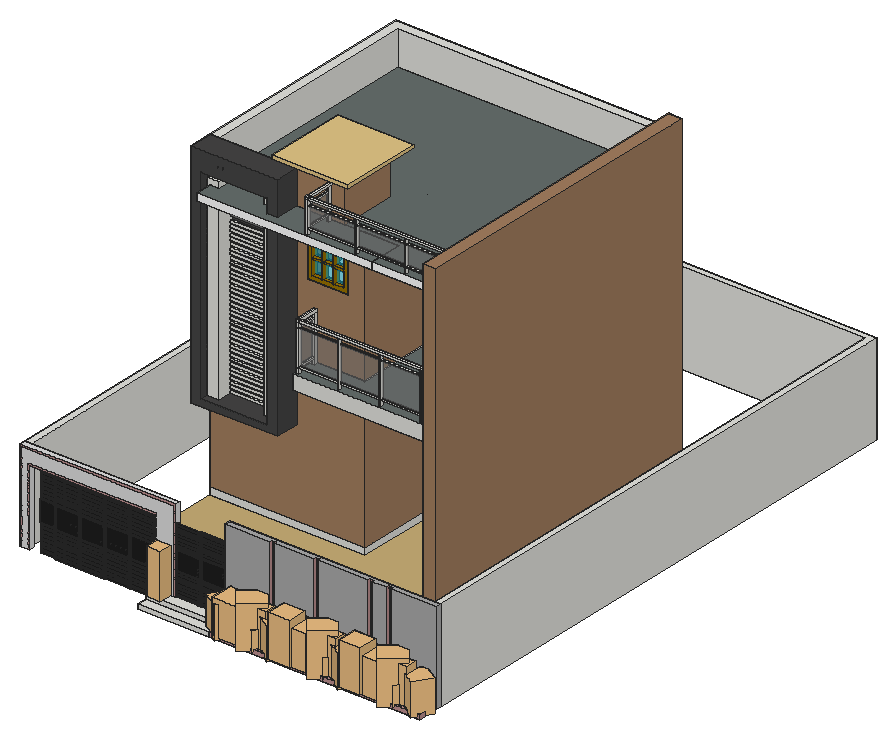
# SketchUp Ruby script. Lengths in inches.
U = 1.inch
M = Sketchup.active_model
def pt(a) = Geom::Point3d.new(a.map { |v| v * U })
def face(e, loops, mat)
  f = e.add_face(loops[0].map { |a| pt(a) })
  loops[1..].each { |l| e.add_face(l.map { |a| pt(a) }).erase! }
  f.material = f.back_material = mat if mat
  f
end
# faces: each face lists its corners as indices into pts; further lists are holes
def faces(e, pts, list, mat = nil) = list.each { |f| face(e, (f[0].is_a?(Array) ? f : [f]).map { |l| l.map { |i| pts[i] } }, mat) }
# xy, xz, yz: faces in a plane at the given z, y or x. An outline is a flat list of corners, or four numbers for a rectangle; further outlines are holes
def ring(l) = l.size == 4 ? [[l[0], l[1]], [l[2], l[1]], [l[2], l[3]], [l[0], l[3]]] : l.each_slice(2).to_a
def flat(e, list, mat, &to3) = list.each { |f| face(e, (f[0].is_a?(Array) ? f : [f]).map { |l| ring(l).map { |u, v| to3.(u, v) } }, mat) }
def xy(e, z, list, mat = nil) = flat(e, list, mat) { |x, y| [x, y, z] }
def xz(e, y, list, mat = nil) = flat(e, list, mat) { |x, z| [x, y, z] }
def yz(e, x, list, mat = nil) = flat(e, list, mat) { |y, z| [x, y, z] }
def lines(e, pts, list) = list.each { |a, b| e.add_line(pt(pts[a]), pt(pts[b])) }
# prism: a flat outline (further loops are holes) pulled along v
def prism(e, loops, v, mat = nil)
  f = face(e, loops, mat); d = Geom::Vector3d.new(v.map { |x| x * U })
  f.pushpull(f.normal.samedirection?(d) ? d.length : -d.length)
end
def box(e, o, s, mat = nil) = prism(e, [[o, [o[0] + s[0], o[1], o[2]], [o[0] + s[0], o[1] + s[1], o[2]], [o[0], o[1] + s[1], o[2]]]], [0, 0, s[2]], mat)
def at(x, y, z, deg = 0) = Geom::Transformation.translation(pt([x, y, z])) * Geom::Transformation.rotation(ORIGIN, Z_AXIS, deg.degrees)
def axes(o, x, y, z) = Geom::Transformation.new([*x, 0, *y, 0, *z, 0, *pt(o).to_a, 1])
def part(name) = M.definitions.add(name)
# library, detail: a bought-in or finely detailed component or shape, given as its bounding box
def library(name, o, s) = part(name).tap { |d| box(d.entities, o, s) }
def detail(e, o, s) = box(e.add_group.entities, o, s)
def put(e, d, t, mat = nil) = e.add_instance(d, t).tap { |i| i.material = mat if mat }
def group(e, t, mat = nil) = e.add_group.tap { |g| g.transformation = t; g.material = mat if mat }.entities
root = M.entities
M.materials.add("Color_008").color = [30, 30, 30]
M.materials.add("Material__1").color = [95, 70, 46]
M.materials.add("[0055_LightGoldenrodYellow]").color = [250, 250, 210]
M.materials.add("[0119_RosyBrown]").color = [188, 143, 143]
M.materials.add("[0130_Gainsboro]").color = [220, 220, 220]
M.materials.add("[0132_LightGray]").color = [169, 169, 169]
M.materials.add("[0134_DimGray]").color = [105, 105, 105]
M.materials.add("[0136_Charcoal]").color = [35, 35, 35]
M.materials.add("[Cladding Siding Tan]").color = [162, 126, 95]
M.materials.add("[Color D07]").color = [153, 114, 0]
M.materials.add("[Color E01]").color = [255, 255, 204]
M.materials.add("[Color M00]").color = [255, 255, 255]
M.materials.add("[Granite Dark Gray]").color = [69, 68, 68]
M.materials.add("[Metal Rusted]").color = [184, 117, 91]
M.materials.add("[Slate]").color = [102, 110, 108]
M.materials.add("[Stone Brushed Khaki]").color = [226, 197, 133]
M.materials.add("[Tile Limestone Multi]").color = [199, 173, 118]
M.materials.add("[Translucent Glass Gray]").color = [128, 128, 128]
M.materials["[Translucent Glass Gray]"].alpha = 0.5
M.materials.add("[Translucent Glass Tinted]").color = [8, 201, 241]
M.materials["[Translucent Glass Tinted]"].alpha = 0.48
M.materials.add("[Wood Bamboo]").color = [177, 105, 43]
M.materials.add("[Wood Floor Parquet]").color = [145, 89, 39]
c1 = part("Frame upright")
box(c1.entities,[0,0,0],[1.9,0.97,93.54])
c2 = part("Vertical picket")
box(c2.entities,[0,0,-2.03],[1.97,0.97,40.94])
c3 = part("Vertical picket \#1")
box(c3.entities,[2.95,0,-2.03],[0.99,0.97,40.94])
c4 = part("Slatted screen panel \#1")
put(c4.entities,c1,axes([87.6,0,0],[1,0,0],[0,1,0],[0,0,0.92593]),"Color_008")
put(c4.entities,c2,axes([48.6875,0,86.61],[0,0,-1],[0,1,0],[1,0,0]),"Color_008")
put(c4.entities,c1,axes([44.75,0,0],[1,0,0],[0,1,0],[0,0,0.92593]),"Color_008")
put(c4.entities,c3,axes([48.6875,0,87.11],[0,0,-1],[0,1,0],[1,0,0]),"[0134_DimGray]")
put(c4.entities,c2,axes([48.6875,0,82.68],[0,0,-1],[0,1,0],[1,0,0]),"Color_008")
put(c4.entities,c3,axes([48.6875,0,83.17],[0,0,-1],[0,1,0],[1,0,0]),"[0134_DimGray]")
put(c4.entities,c3,axes([48.6875,0,75.3],[0,0,-1],[0,1,0],[1,0,0]),"[0134_DimGray]")
put(c4.entities,c2,axes([48.6875,0,78.74],[0,0,-1],[0,1,0],[1,0,0]),"Color_008")
put(c4.entities,c2,axes([48.6875,0,74.8],[0,0,-1],[0,1,0],[1,0,0]),"Color_008")
put(c4.entities,c3,axes([48.6875,0,79.23],[0,0,-1],[0,1,0],[1,0,0]),"[0134_DimGray]")
put(c4.entities,c3,axes([48.6875,0,67.42],[0,0,-1],[0,1,0],[1,0,0]),"[0134_DimGray]")
put(c4.entities,c3,axes([48.6875,0,71.36],[0,0,-1],[0,1,0],[1,0,0]),"[0134_DimGray]")
put(c4.entities,c2,axes([48.6875,0,70.87],[0,0,-1],[0,1,0],[1,0,0]),"Color_008")
put(c4.entities,c2,axes([48.6875,0,66.93],[0,0,-1],[0,1,0],[1,0,0]),"Color_008")
put(c4.entities,c2,axes([48.6875,0,59.06],[0,0,-1],[0,1,0],[1,0,0]),"Color_008")
put(c4.entities,c2,axes([48.6875,0,62.99],[0,0,-1],[0,1,0],[1,0,0]),"Color_008")
put(c4.entities,c3,axes([48.6875,0,59.55],[0,0,-1],[0,1,0],[1,0,0]),"[0134_DimGray]")
put(c4.entities,c3,axes([48.6875,0,63.48],[0,0,-1],[0,1,0],[1,0,0]),"[0134_DimGray]")
put(c4.entities,c3,axes([48.6875,0,33.96],[0,0,-1],[0,1,0],[1,0,0]),"[0134_DimGray]")
put(c4.entities,c2,axes([48.6875,0,29.53],[0,0,-1],[0,1,0],[1,0,0]),"Color_008")
put(c4.entities,c3,axes([48.6875,0,30.02],[0,0,-1],[0,1,0],[1,0,0]),"[0134_DimGray]")
put(c4.entities,c2,axes([48.6875,0,25.59],[0,0,-1],[0,1,0],[1,0,0]),"Color_008")
put(c4.entities,c2,axes([48.6875,0,33.46],[0,0,-1],[0,1,0],[1,0,0]),"Color_008")
put(c4.entities,c3,axes([48.6875,0,26.08],[0,0,-1],[0,1,0],[1,0,0]),"[0134_DimGray]")
put(c4.entities,c2,axes([48.6875,0,13.78],[0,0,-1],[0,1,0],[1,0,0]),"Color_008")
put(c4.entities,c3,axes([48.6875,0,10.33],[0,0,-1],[0,1,0],[1,0,0]),"[0134_DimGray]")
put(c4.entities,c2,axes([48.6875,0,21.65],[0,0,-1],[0,1,0],[1,0,0]),"Color_008")
put(c4.entities,c2,axes([48.6875,0,5.91],[0,0,-1],[0,1,0],[1,0,0]),"Color_008")
put(c4.entities,c3,axes([48.6875,0,22.15],[0,0,-1],[0,1,0],[1,0,0]),"[0134_DimGray]")
put(c4.entities,c2,axes([48.6875,0,1.97],[0,0,-1],[0,1,0],[1,0,0]),"Color_008")
put(c4.entities,c2,axes([48.6875,0,9.84],[0,0,-1],[0,1,0],[1,0,0]),"Color_008")
put(c4.entities,c3,axes([48.6875,0,6.4],[0,0,-1],[0,1,0],[1,0,0]),"[0134_DimGray]")
put(c4.entities,c3,axes([48.6875,0,18.21],[0,0,-1],[0,1,0],[1,0,0]),"[0134_DimGray]")
put(c4.entities,c2,axes([48.6875,0,17.72],[0,0,-1],[0,1,0],[1,0,0]),"Color_008")
put(c4.entities,c3,axes([48.6875,0,14.27],[0,0,-1],[0,1,0],[1,0,0]),"[0134_DimGray]")
put(c4.entities,c2,axes([48.6875,0,49.7],[0,0,-1],[0,1,0],[1,0,0]),"Color_008")
put(c4.entities,c2,axes([48.6875,0,44.29],[0,0,-1],[0,1,0],[1,0,0]),"Color_008")
put(c4.entities,c2,axes([48.6875,0,38.88],[0,0,-1],[0,1,0],[1,0,0]),"Color_008")
put(c4.entities,c2,axes([48.6875,0,55.12],[0,0,-1],[0,1,0],[1,0,0]),"Color_008")
c5 = part("Infill panel")
box(c5.entities,[0,0,-1.97],[52.81,0.39,23.62])
c6 = part("Slatted screen panel")
p = [[42.85,0.97,43.31],[42.85,0.97,44.29]]
lines(c6.entities,p,[[0,1]])
put(c6.entities,c2,axes([3.9375,0,86.61],[0,0,-1],[0,1,0],[1,0,0]),"Color_008")
put(c6.entities,c1,axes([87.6,0,0],[1,0,0],[0,1,0],[0,0,0.92593]),"Color_008")
put(c6.entities,c2,axes([48.6875,0,86.61],[0,0,-1],[0,1,0],[1,0,0]),"Color_008")
put(c6.entities,c1,axes([0,0,0],[1,0,0],[0,1,0],[0,0,0.92593]),"Color_008")
put(c6.entities,c1,axes([42.85,0,0],[1,0,0],[0,1,0],[0,0,0.92593]),"Color_008")
put(c6.entities,c1,axes([44.75,0,0],[1,0,0],[0,1,0],[0,0,0.92593]),"Color_008")
put(c6.entities,c3,axes([3.9375,0,87.11],[0,0,-1],[0,1,0],[1,0,0]),"[0134_DimGray]")
put(c6.entities,c3,axes([48.6875,0,87.11],[0,0,-1],[0,1,0],[1,0,0]),"[0134_DimGray]")
put(c6.entities,c2,axes([48.6875,0,82.68],[0,0,-1],[0,1,0],[1,0,0]),"Color_008")
put(c6.entities,c3,axes([48.6875,0,83.17],[0,0,-1],[0,1,0],[1,0,0]),"[0134_DimGray]")
put(c6.entities,c3,axes([3.9375,0,83.17],[0,0,-1],[0,1,0],[1,0,0]),"[0134_DimGray]")
put(c6.entities,c2,axes([3.9375,0,82.68],[0,0,-1],[0,1,0],[1,0,0]),"Color_008")
put(c6.entities,c3,axes([48.6875,0,75.3],[0,0,-1],[0,1,0],[1,0,0]),"[0134_DimGray]")
put(c6.entities,c2,axes([48.6875,0,78.74],[0,0,-1],[0,1,0],[1,0,0]),"Color_008")
put(c6.entities,c2,axes([48.6875,0,74.8],[0,0,-1],[0,1,0],[1,0,0]),"Color_008")
put(c6.entities,c3,axes([48.6875,0,79.23],[0,0,-1],[0,1,0],[1,0,0]),"[0134_DimGray]")
put(c6.entities,c3,axes([3.9375,0,75.3],[0,0,-1],[0,1,0],[1,0,0]),"[0134_DimGray]")
put(c6.entities,c2,axes([3.9375,0,78.74],[0,0,-1],[0,1,0],[1,0,0]),"Color_008")
put(c6.entities,c3,axes([3.9375,0,79.23],[0,0,-1],[0,1,0],[1,0,0]),"[0134_DimGray]")
put(c6.entities,c2,axes([3.9375,0,74.8],[0,0,-1],[0,1,0],[1,0,0]),"Color_008")
put(c6.entities,c3,axes([48.6875,0,67.42],[0,0,-1],[0,1,0],[1,0,0]),"[0134_DimGray]")
put(c6.entities,c3,axes([3.9375,0,63.48],[0,0,-1],[0,1,0],[1,0,0]),"[0134_DimGray]")
put(c6.entities,c3,axes([48.6875,0,71.36],[0,0,-1],[0,1,0],[1,0,0]),"[0134_DimGray]")
put(c6.entities,c3,axes([3.9375,0,67.42],[0,0,-1],[0,1,0],[1,0,0]),"[0134_DimGray]")
put(c6.entities,c2,axes([3.9375,0,70.87],[0,0,-1],[0,1,0],[1,0,0]),"Color_008")
put(c6.entities,c2,axes([48.6875,0,70.87],[0,0,-1],[0,1,0],[1,0,0]),"Color_008")
put(c6.entities,c2,axes([48.6875,0,66.93],[0,0,-1],[0,1,0],[1,0,0]),"Color_008")
put(c6.entities,c2,axes([48.6875,0,59.06],[0,0,-1],[0,1,0],[1,0,0]),"Color_008")
put(c6.entities,c2,axes([3.9375,0,55.12],[0,0,-1],[0,1,0],[1,0,0]),"Color_008")
put(c6.entities,c2,axes([3.9375,0,62.99],[0,0,-1],[0,1,0],[1,0,0]),"Color_008")
put(c6.entities,c3,axes([3.9375,0,59.55],[0,0,-1],[0,1,0],[1,0,0]),"[0134_DimGray]")
put(c6.entities,c2,axes([3.9375,0,66.93],[0,0,-1],[0,1,0],[1,0,0]),"Color_008")
put(c6.entities,c2,axes([48.6875,0,62.99],[0,0,-1],[0,1,0],[1,0,0]),"Color_008")
put(c6.entities,c3,axes([48.6875,0,59.55],[0,0,-1],[0,1,0],[1,0,0]),"[0134_DimGray]")
put(c6.entities,c3,axes([48.6875,0,63.48],[0,0,-1],[0,1,0],[1,0,0]),"[0134_DimGray]")
put(c6.entities,c2,axes([3.9375,0,59.06],[0,0,-1],[0,1,0],[1,0,0]),"Color_008")
put(c6.entities,c3,axes([3.9375,0,71.36],[0,0,-1],[0,1,0],[1,0,0]),"[0134_DimGray]")
put(c6.entities,c3,axes([3.9375,0,33.96],[0,0,-1],[0,1,0],[1,0,0]),"[0134_DimGray]")
put(c6.entities,c3,axes([48.6875,0,33.96],[0,0,-1],[0,1,0],[1,0,0]),"[0134_DimGray]")
put(c6.entities,c2,axes([3.9375,0,29.53],[0,0,-1],[0,1,0],[1,0,0]),"Color_008")
put(c6.entities,c3,axes([3.9375,0,26.08],[0,0,-1],[0,1,0],[1,0,0]),"[0134_DimGray]")
put(c6.entities,c2,axes([3.9375,0,33.46],[0,0,-1],[0,1,0],[1,0,0]),"Color_008")
put(c6.entities,c2,axes([48.6875,0,29.53],[0,0,-1],[0,1,0],[1,0,0]),"Color_008")
put(c6.entities,c3,axes([48.6875,0,30.02],[0,0,-1],[0,1,0],[1,0,0]),"[0134_DimGray]")
put(c6.entities,c2,axes([3.9375,0,25.59],[0,0,-1],[0,1,0],[1,0,0]),"Color_008")
put(c6.entities,c2,axes([48.6875,0,25.59],[0,0,-1],[0,1,0],[1,0,0]),"Color_008")
put(c6.entities,c2,axes([48.6875,0,33.46],[0,0,-1],[0,1,0],[1,0,0]),"Color_008")
put(c6.entities,c2,axes([3.9375,0,49.7],[0,0,-1],[0,1,0],[1,0,0]),"Color_008")
put(c6.entities,c3,axes([48.6875,0,26.08],[0,0,-1],[0,1,0],[1,0,0]),"[0134_DimGray]")
put(c6.entities,c3,axes([3.9375,0,30.02],[0,0,-1],[0,1,0],[1,0,0]),"[0134_DimGray]")
put(c6.entities,c2,axes([3.9375,0,5.91],[0,0,-1],[0,1,0],[1,0,0]),"Color_008")
put(c6.entities,c2,axes([48.6875,0,13.78],[0,0,-1],[0,1,0],[1,0,0]),"Color_008")
put(c6.entities,c3,axes([48.6875,0,10.33],[0,0,-1],[0,1,0],[1,0,0]),"[0134_DimGray]")
put(c6.entities,c3,axes([3.9375,0,6.4],[0,0,-1],[0,1,0],[1,0,0]),"[0134_DimGray]")
put(c6.entities,c2,axes([3.9375,0,13.78],[0,0,-1],[0,1,0],[1,0,0]),"Color_008")
put(c6.entities,c2,axes([48.6875,0,21.65],[0,0,-1],[0,1,0],[1,0,0]),"Color_008")
put(c6.entities,c2,axes([48.6875,0,5.91],[0,0,-1],[0,1,0],[1,0,0]),"Color_008")
put(c6.entities,c3,axes([48.6875,0,22.15],[0,0,-1],[0,1,0],[1,0,0]),"[0134_DimGray]")
put(c6.entities,c2,axes([48.6875,0,1.97],[0,0,-1],[0,1,0],[1,0,0]),"Color_008")
put(c6.entities,c2,axes([48.6875,0,9.84],[0,0,-1],[0,1,0],[1,0,0]),"Color_008")
put(c6.entities,c3,axes([48.6875,0,6.4],[0,0,-1],[0,1,0],[1,0,0]),"[0134_DimGray]")
put(c6.entities,c2,axes([3.9375,0,9.84],[0,0,-1],[0,1,0],[1,0,0]),"Color_008")
put(c6.entities,c3,axes([3.9375,0,10.33],[0,0,-1],[0,1,0],[1,0,0]),"[0134_DimGray]")
put(c6.entities,c3,axes([3.9375,0,22.15],[0,0,-1],[0,1,0],[1,0,0]),"[0134_DimGray]")
put(c6.entities,c2,axes([3.9375,0,1.97],[0,0,-1],[0,1,0],[1,0,0]),"Color_008")
put(c6.entities,c3,axes([3.9375,0,18.21],[0,0,-1],[0,1,0],[1,0,0]),"[0134_DimGray]")
put(c6.entities,c3,axes([3.9375,0,14.27],[0,0,-1],[0,1,0],[1,0,0]),"[0134_DimGray]")
put(c6.entities,c2,axes([3.9375,0,21.65],[0,0,-1],[0,1,0],[1,0,0]),"Color_008")
put(c6.entities,c3,axes([48.6875,0,18.21],[0,0,-1],[0,1,0],[1,0,0]),"[0134_DimGray]")
put(c6.entities,c2,axes([3.9375,0,17.72],[0,0,-1],[0,1,0],[1,0,0]),"Color_008")
put(c6.entities,c2,axes([48.6875,0,17.72],[0,0,-1],[0,1,0],[1,0,0]),"Color_008")
put(c6.entities,c3,axes([48.6875,0,14.27],[0,0,-1],[0,1,0],[1,0,0]),"[0134_DimGray]")
put(c6.entities,c2,axes([3.9375,0,44.29],[0,0,-1],[0,1,0],[1,0,0]),"Color_008")
put(c6.entities,c2,axes([3.9375,0,38.88],[0,0,-1],[0,1,0],[1,0,0]),"Color_008")
put(c6.entities,c2,axes([48.6875,0,49.7],[0,0,-1],[0,1,0],[1,0,0]),"Color_008")
put(c6.entities,c2,axes([48.6875,0,44.29],[0,0,-1],[0,1,0],[1,0,0]),"Color_008")
put(c6.entities,c2,axes([48.6875,0,38.88],[0,0,-1],[0,1,0],[1,0,0]),"Color_008")
put(c6.entities,c2,axes([48.6875,0,55.12],[0,0,-1],[0,1,0],[1,0,0]),"Color_008")
c7 = part("Group\#19")
put(c7.entities,c5,axes([0,0,33.46],[0.82011,0,0],[0,1,0],[0,0,1]),"Color_008")
put(c7.entities,c6,axes([0,0.39,0],[0.96774,0,0],[0,1,0],[0,0,1]),"[0055_LightGoldenrodYellow]")
put(c7.entities,c5,axes([43.31,0,33.46],[0.82011,0,0],[0,1,0],[0,0,1]),"Color_008")
c8 = library("Areca palm plant",[0,0,0],[49.1,36.6,54.46])
c9 = library("Group\#74",[-84.69,-90.07,-0.36],[176.51,175.13,171.4])
c10 = library("Group\#130",[-7.34,-1.2,0],[38.67,35.81,49.04])
c11 = library("Group38\#2",[14.01,28.44,-23.43],[18.58,18.32,38.89])
c12 = library("Group20\#1",[-20.81,-17.08,3.79],[39.86,39.43,37.51])
c13 = library("Group\#39",[0,0,0],[39.23,38.16,78.77])
c14 = part("compound +++")
g1 = group(c14.entities,at(40.59,15.26,0))
g2 = group(g1,at(295.3,30.86,0),"[0132_LightGray]")
xy(g2,0,[[0,0,304.7,8]])
xy(g2,9,[[205.47,0,211.47,3]],"[0119_RosyBrown]")
xy(g2,9,[[64.54,0,70.54,3],[127.35,0,133.35,3],[232.97,0,238.97,3]],"[0136_Charcoal]")
xy(g2,84,[[0,0,64.54,0,64.54,3,70.54,3,70.54,0,127.35,0,127.35,3,133.35,3,133.35,0,205.47,0,205.47,3,211.47,3,211.47,0,232.97,0,232.97,3,238.97,3,238.97,0,304.7,0,304.7,8,0,8],[232.97,0,238.97,3]])
xz(g2,0,[[0,0,304.7,0,304.7,84,238.97,84,238.97,9,232.97,9,232.97,84,211.47,84,211.47,9,205.47,9,205.47,84,133.35,84,133.35,9,127.35,9,127.35,84,70.54,84,70.54,9,64.54,9,64.54,84,0,84]])
xz(g2,3,[[64.54,9,70.54,84],[127.35,9,133.35,84],[205.47,9,211.47,84],[232.97,9,238.97,84]],"[0119_RosyBrown]")
xz(g2,8,[[0,0,304.7,84]])
yz(g2,0,[[0,0,8,84]])
yz(g2,64.54,[[0,9,3,84]],"[0119_RosyBrown]")
yz(g2,70.54,[[0,9,3,84]],"[0119_RosyBrown]")
yz(g2,127.35,[[0,9,3,84]],"[0119_RosyBrown]")
yz(g2,133.35,[[0,9,3,84]],"[0119_RosyBrown]")
yz(g2,205.47,[[0,9,3,84]],"[0119_RosyBrown]")
yz(g2,211.47,[[0,9,3,84]],"[0119_RosyBrown]")
yz(g2,232.97,[[0,9,3,84]],"[0119_RosyBrown]")
yz(g2,238.97,[[0,9,3,84]],"[0119_RosyBrown]")
yz(g2,304.7,[[0,0,8,84]])
g3 = group(g1,at(0,30.86,0),"[0130_Gainsboro]")
xy(g3,0,[[0,0,13.34,8],[193.34,0,223.34,8]])
xy(g3,69,[[13.34,0,193.34,8]])
xy(g3,84,[[0,0,223.34,8]])
xz(g3,0,[[2,0,11.34,0,11.34,71,195.34,71,195.34,0,221.34,0,221.34,82,2,82]])
xz(g3,0,[[0,0,2,0,2,82,221.34,82,221.34,0,223.34,0,223.34,84,0,84],[11.34,0,13.34,0,13.34,69,193.34,69,193.34,0,195.34,0,195.34,71,11.34,71]],"[0119_RosyBrown]")
xz(g3,8,[[0,0,0,84,223.34,84,223.34,0,193.34,0,193.34,69,13.34,69,13.34,0]])
yz(g3,0,[[0,0,8,84]])
yz(g3,13.34,[[0,0,8,69]])
yz(g3,193.34,[[0,0,8,69]])
yz(g3,223.34,[[0,0,8,84]])
g4 = group(g1,at(13.34,31.16,0))
g5 = group(g4,at(13.67,1.64,0))
put(g5,c4,axes([-35.99,0.33,0],[0.80418,0,0],[0,0.83,0],[0,0,0.79664]),"[0055_LightGoldenrodYellow]")
put(g5,c5,axes([0,0,26.66],[0.68149,0,0],[0,0.83,0],[0,0,0.79664]),"Color_008")
g6 = group(g4,at(35.99,0,0))
put(g6,c7,axes([0,0,0],[0.83098,0,0],[0,0.83,0],[0,0,0.79664]))
put(g6,c7,axes([71.97,0,0],[0.83098,0,0],[0,0.83,0],[0,0,0.79664]))
put(g1,c7,axes([223.34,31.16,8],[0.83,0,0],[0,0.83,0],[0,0,0.70427]))
g7 = group(g1,at(193.34,15.86,4))
prism(g7,[[[0,0,0],[0,15,0],[30,15,0],[30,23,0],[101.95,23,0],[101.95,0,0]]],[0,0,4])
g8 = group(g1,at(193.34,-6.89,0))
prism(g8,[[[0,37.75,0],[30,37.75,0],[30,45.75,0],[101.95,45.75,0],[101.95,7.75,0],[0,7.75,0]]],[0,0,4])
g9 = group(g1,at(295.3,15.86,0),"[0119_RosyBrown]")
xy(g9,0,[[0,-15,304.7,15]])
xy(g9,0.5625,[[3,-12,301.7,12]])
xy(g9,4,[[[0,-15,304.7,15],[3,-12,301.7,12]]])
xz(g9,-15,[[0,0,304.7,4]])
xz(g9,-12,[[3,0.5625,301.7,4]])
xz(g9,12,[[3,0.5625,301.7,4]])
xz(g9,15,[[0,0,304.7,4]])
yz(g9,0,[[-15,0,15,4]])
yz(g9,3,[[-12,0.5625,12,4]])
yz(g9,301.7,[[-12,0.5625,12,4]])
yz(g9,304.7,[[-15,0,15,4]])
g10 = group(g1,at(600.32,0,1.05,90))
put(g10,c8,axes([-8.34,156.73,0.03],[0.45017,-0.56191,0],[0.66137,0.52986,0],[0,0,0.72]))
put(g10,c8,axes([-8.34,54.91,0.03],[0.45017,-0.56191,0],[0.66137,0.52986,0],[0,0,0.72]))
put(g10,c8,axes([-8.34,257.79,0.03],[0.45017,-0.56191,0],[0.66137,0.52986,0],[0,0,0.72]))
put(g10,c9,axes([15.05,119.55,0.03],[-0.08133,-0.14087,0],[0.14087,-0.08133,0],[0,0,0.1725]))
put(g10,c10,axes([22.79,88.23,1.95],[0,0.79,0],[-0.79,0,0],[0,0,0.79]))
put(g10,c9,axes([12.79,69.62,0],[-0.04961,-0.08593,0],[0.08593,-0.04961,0],[0,0,0.10522]))
put(g10,c9,axes([15.05,221.36,0.03],[-0.08133,-0.14087,0],[0.14087,-0.08133,0],[0,0,0.1725]))
put(g10,c10,axes([22.79,190.04,1.95],[0,0.79,0],[-0.79,0,0],[0,0,0.79]))
put(g10,c11,axes([-6.25,98.98,22.125],[0.8848,0,0],[0,0.94674,0],[0,0,0.85826]))
put(g10,c11,axes([-6.25,-2.84,22.125],[0.8848,0,0],[0,0.94674,0],[0,0,0.85826]))
put(g10,c9,axes([15.05,14.11,0.03],[-0.08133,-0.14087,0],[0.14087,-0.08133,0],[0,0,0.1725]))
g11 = group(g10,at(-2.14,-1.68,-6.05))
xy(g11,7,[[6,5,30,303.7]],"Material__1")
put(g10,c9,axes([12.79,144.18,0],[-0.04961,-0.08593,0],[0.08593,-0.04961,0],[0,0,0.10522]))
put(g10,c9,axes([12.79,42.37,0],[-0.04961,-0.08593,0],[0.08593,-0.04961,0],[0,0,0.10522]))
put(g10,c9,axes([12.79,191.5,0],[-0.04961,-0.08593,0],[0.08593,-0.04961,0],[0,0,0.10522]))
put(g10,c12,axes([16.82,180.11,-1.27],[0,0.85,0],[-0.85,0,0],[0,0,0.85]))
put(g10,c9,axes([12.79,171.43,0],[-0.04961,-0.08593,0],[0.08593,-0.04961,0],[0,0,0.10522]))
put(g10,c12,axes([16.82,78.29,-1.27],[0,0.85,0],[-0.85,0,0],[0,0,0.85]))
put(g10,c9,axes([12.79,89.68,0],[-0.04961,-0.08593,0],[0.08593,-0.04961,0],[0,0,0.10522]))
put(g10,c9,axes([12.79,245.25,0],[-0.04961,-0.08593,0],[0.08593,-0.04961,0],[0,0,0.10522]))
put(g10,c9,axes([12.79,272.5,0],[-0.04961,-0.08593,0],[0.08593,-0.04961,0],[0,0,0.10522]))
put(g10,c12,axes([16.82,281.17,-1.27],[0,0.85,0],[-0.85,0,0],[0,0,0.85]))
put(g10,c11,axes([-6.25,200.04,22.125],[0.8848,0,0],[0,0.94674,0],[0,0,0.85826]))
put(g10,c9,axes([15.05,296.8,0.03],[-0.08133,-0.14087,0],[0.14087,-0.08133,0],[0,0,0.1725]))
put(g1,c13,axes([216.59,12.0625,8],[0,0.52198,0],[-0.52198,0,0],[0,0,0.52198]),"[0134_DimGray]")
c15 = part("Difference\#1")
xy(c15.entities,0,[[[0,0,0,207,243,207,243,69,138,69,138,0],[9,9,129,9,129,78,234,78,234,198,9,198]]])
xy(c15.entities,3,[[147.38,69,184.09,78]])
xy(c15.entities,42.375,[[189.1,69,232.6,78]])
xy(c15.entities,85.875,[[189.1,69,232.6,78]])
xy(c15.entities,86,[[147.38,69,184.09,78]])
xy(c15.entities,120,[[[0,0,138,0,138,69,243,69,243,207,0,207],[9,9,9,198,234,198,234,78,129,78,129,9]]])
xz(c15.entities,0,[[0,0,138,120]])
xz(c15.entities,9,[[9,0,129,120]])
xz(c15.entities,69,[[[138,0,243,120],[147.38,3,184.09,86],[189.1,42.375,232.6,85.875]]],"[Metal Rusted]")
xz(c15.entities,78,[[[129,0,234,120],[147.38,3,184.09,86],[189.1,42.375,232.6,85.875]]])
xz(c15.entities,198,[[9,0,234,120]])
xz(c15.entities,207,[[0,0,243,120]])
yz(c15.entities,0,[[0,0,207,120]])
yz(c15.entities,9,[[9,0,198,120]])
yz(c15.entities,129,[[9,0,78,120]])
yz(c15.entities,138,[[0,0,69,120]])
yz(c15.entities,147.38,[[69,3,78,86]])
yz(c15.entities,184.09,[[69,3,78,86]])
yz(c15.entities,189.1,[[69,42.375,78,85.875]])
yz(c15.entities,232.6,[[69,42.375,78,85.875]])
yz(c15.entities,234,[[78,0,198,120]])
yz(c15.entities,243,[[69,0,207,120]])
c16 = library("Group\#3",[0,0,0],[36.71,10.47,83])
c17 = part("Group11\#1")
xy(c17.entities,0,[[-17.8125,-17.8125,-6.73,17.8125],[-5.54,-17.8125,5.54,17.8125],[6.73,-17.8125,17.8125,17.8125]])
c18 = part("Group10\#1")
xy(c18.entities,0,[[[-21.75,-21.75,21.75,21.75],[6.73,-17.8125,17.8125,17.8125],[-17.8125,-17.8125,-6.73,17.8125],[-5.54,-17.8125,5.54,17.8125]]])
xy(c18.entities,5.875,[[[-21.75,-21.75,21.75,21.75],[6.73,-17.8125,17.8125,17.8125],[-17.8125,-17.8125,-6.73,17.8125],[-5.54,-17.8125,5.54,17.8125]]],"[Wood Floor Parquet]")
xz(c18.entities,-21.75,[[-21.75,0,21.75,5.875]])
xz(c18.entities,-17.8125,[[-17.8125,0,-6.73,5.875]],"[Wood Bamboo]")
xz(c18.entities,-17.8125,[[-5.54,0,5.54,5.875],[6.73,0,17.8125,5.875]],"[Wood Floor Parquet]")
xz(c18.entities,17.8125,[[-17.8125,0,-6.73,5.875],[-5.54,0,5.54,5.875],[6.73,0,17.8125,5.875]],"[Wood Floor Parquet]")
xz(c18.entities,21.75,[[-21.75,0,21.75,5.875]])
yz(c18.entities,-21.75,[[-21.75,0,21.75,5.875]])
yz(c18.entities,-17.8125,[[-17.8125,0,17.8125,5.875]],"[Wood Floor Parquet]")
yz(c18.entities,-6.73,[[-17.8125,0,17.8125,5.875]],"[Wood Floor Parquet]")
yz(c18.entities,-5.54,[[-17.8125,0,17.8125,5.875]],"[Wood Floor Parquet]")
yz(c18.entities,5.54,[[-17.8125,0,17.8125,5.875]],"[Wood Floor Parquet]")
yz(c18.entities,6.73,[[-17.8125,0,17.8125,5.875]],"[Wood Floor Parquet]")
yz(c18.entities,17.8125,[[-17.8125,0,17.8125,5.875]],"[Wood Floor Parquet]")
yz(c18.entities,21.75,[[-21.75,0,21.75,5.875]])
put(c18.entities,c17,at(0,0,2.9375),"[Translucent Glass Tinted]")
c19 = part("Group3\#2")
p = [[737.1,1857.0625,42.375],[737.1,1857.0625,85.875],[780.6,1857.0625,85.875],[780.6,1857.0625,42.375]]
lines(c19.entities,p,[[0,1],[1,2],[2,3],[3,0]])
g12 = group(c19.entities,at(548,1788.0625,0))
put(g12,c15,at(0,0,0))
put(g12,c16,at(147.38,67.53,3))
put(c19.entities,c18,axes([758.85,1862.9375,64.125],[1,0,0],[0,0,1],[0,-1,0]))
c20 = part("Difference")
xy(c20.entities,0,[[[0,0,0,207,243,207,243,69,138,69,138,0],[9,9,129,9,129,78,234,78,234,198,9,198]]])
xy(c20.entities,3,[[147.38,69,184.09,78]])
xy(c20.entities,42.375,[[189.1,69,232.6,78]])
xy(c20.entities,70.6,[[86.81,0,122.81,9]])
xy(c20.entities,85.875,[[189.1,69,232.6,78]])
xy(c20.entities,86,[[147.38,69,184.09,78]])
xy(c20.entities,106.6,[[86.81,0,122.81,9]])
xy(c20.entities,120,[[[0,0,138,0,138,69,243,69,243,207,0,207],[9,9,9,198,234,198,234,78,129,78,129,9]]])
xz(c20.entities,0,[[[0,0,138,120],[86.81,70.6,122.81,106.6]]])
xz(c20.entities,9,[[[9,0,129,120],[86.81,70.6,122.81,106.6]]])
xz(c20.entities,69,[[[138,0,243,120],[147.38,3,184.09,86],[189.1,42.375,232.6,85.875]]],"[Metal Rusted]")
xz(c20.entities,78,[[[129,0,234,120],[147.38,3,184.09,86],[189.1,42.375,232.6,85.875]]])
xz(c20.entities,198,[[9,0,234,120]])
xz(c20.entities,207,[[0,0,243,120]])
yz(c20.entities,0,[[0,0,207,120]])
yz(c20.entities,9,[[9,0,198,120]])
yz(c20.entities,86.81,[[0,70.6,9,106.6]])
yz(c20.entities,122.81,[[0,70.6,9,106.6]])
yz(c20.entities,129,[[9,0,78,120]])
yz(c20.entities,138,[[0,0,69,120]])
yz(c20.entities,147.38,[[69,3,78,86]])
yz(c20.entities,184.09,[[69,3,78,86]])
yz(c20.entities,189.1,[[69,42.375,78,85.875]])
yz(c20.entities,232.6,[[69,42.375,78,85.875]])
yz(c20.entities,234,[[78,0,198,120]])
yz(c20.entities,243,[[69,0,207,120]])
c21 = part("Group3\#1")
p = [[737.1,1857.0625,42.375],[737.1,1857.0625,85.875],[780.6,1857.0625,85.875],[780.6,1857.0625,42.375]]
lines(c21.entities,p,[[0,1],[1,2],[2,3],[3,0]])
g13 = group(c21.entities,at(548,1788.0625,0))
put(g13,c20,at(0,0,0))
put(g13,c16,at(147.38,67.53,3))
put(c21.entities,c18,axes([758.85,1862.9375,64.125],[1,0,0],[0,0,1],[0,-1,0]))
c22 = part("Group\#10")
prism(c22.entities,[[[0,0.625,0.3125],[0,0.61,0.23],[0,0.58,0.16],[0,0.53,0.09],[0,0.47,0.04],[0,0.39,0.01],[0,0.3125,0],[0,0.23,0.01],[0,0.16,0.04],[0,0.09,0.09],[0,0.04,0.16],[0,0.01,0.23],[0,0,0.3125],[0,0.01,0.39],[0,0.04,0.47],[0,0.09,0.53],[0,0.16,0.58],[0,0.23,0.61],[0,0.3125,0.625],[0,0.39,0.61],[0,0.47,0.58],[0,0.53,0.53],[0,0.58,0.47],[0,0.61,0.39]]],[59.09,0,0])
c23 = part("Group\#11")
yz(c23.entities,0,[[0.3125,0,0.39,0.01,0.47,0.04,0.53,0.09,0.58,0.16,0.61,0.23,0.625,0.3125,0.61,0.39,0.58,0.47,0.53,0.53,0.47,0.58,0.39,0.61,0.3125,0.625,0.23,0.61,0.16,0.58,0.09,0.53,0.04,0.47,0.01,0.39,0,0.3125,0.01,0.23,0.04,0.16,0.09,0.09,0.16,0.04,0.23,0.01]])
c24 = part("Group\#18")
box(c24.entities,[0,-2,0],[38.34,2,2.32])
c25 = part("Group27\#1")
box(c25.entities,[641.63,1784.34,133.1875],[2.37,2.36,41.54])
c26 = part("Group28\#1")
box(c26.entities,[641.63,1766.65,133.1875],[2.37,2.36,41.54])
c27 = part("Group30\#1")
box(c27.entities,[641.4375,1766.65,174.73],[2.75,20.05,1.77])
c28 = part("Group30\#2")
box(c28.entities,[641.83,1767.83,169.61],[1.97,17.69,0.98])
c29 = part("Group31\#1")
box(c29.entities,[641.83,1767.83,138.11],[1.97,17.69,0.98])
c30 = part("Group32\#1")
yz(c30.entities,642.8125,[[1767.83,139.09,1785.52,169.61]])
c31 = part("Group34\#2")
box(c31.entities,[788.51,1766.65,133.1875],[2.36,2.36,41.54])
c32 = part("Group35\#1")
box(c32.entities,[678.94,1766.65,133.1875],[1.18,2.36,41.54])
box(c32.entities,[715.66,1766.65,133.1875],[1.18,2.36,41.54])
box(c32.entities,[752.38,1766.65,133.1875],[1.18,2.36,41.54])
c33 = part("Group36\#1")
box(c33.entities,[641.63,1766.46,174.73],[149.24,2.75,1.77])
c34 = part("Group37\#1")
box(c34.entities,[642.8125,1766.85,169.61],[146.875,1.97,0.98])
c35 = part("Group38\#1")
box(c35.entities,[642.8125,1766.85,138.11],[146.875,1.97,0.98])
c36 = part("Group39\#1")
xz(c36.entities,1767.83,[[642.8125,139.09,789.6875,169.61]],"[Translucent Glass Gray]")
c37 = part("Group59\#1")
box(c37.entities,[654.99,1783.97,252],[2.36,2.36,28.23])
c38 = part("Group60\#1")
box(c38.entities,[654.99,1759.85,252],[2.36,2.36,28.23])
c39 = part("Group62\#1")
box(c39.entities,[654.79,1759.85,280.23],[2.76,26.48,1.77])
c40 = part("Group62\#2")
box(c40.entities,[655.1875,1761.03,275.11],[1.96,24.12,0.98])
c41 = part("Group63\#1")
box(c41.entities,[655.1875,1761.03,256.92],[1.96,24.12,0.99])
c42 = part("Group64\#1")
yz(c42.entities,656.17,[[1761.03,257.91,1785.15,275.11]])
c43 = part("Group66\#2")
box(c43.entities,[787.43,1759.85,252],[2.36,2.36,28.23])
c44 = part("Group67\#1")
box(c44.entities,[699.73,1759.85,252],[1.18,2.36,28.23])
box(c44.entities,[743.87,1759.85,252],[1.18,2.36,28.23])
c45 = part("Group68\#1")
box(c45.entities,[654.99,1759.65,280.23],[134.8,2.76,1.77])
c46 = part("Group69\#1")
box(c46.entities,[656.17,1760.04,275.11],[132.44,1.97,0.98])
c47 = part("Group70\#1")
box(c47.entities,[656.17,1760.04,256.92],[132.44,1.97,0.99])
c48 = part("Group71\#1")
xz(c48.entities,1761.03,[[656.17,257.91,788.61,275.11]])
c49 = part("Group72\#1")
prism(c49.entities,[[[791,1995.0625,252],[791,1986.0625,252],[557,1986.0625,252],[557,1788.0625,252],[548,1788.0625,252],[548,1995.0625,252]]],[0,0,30])
c50 = part("Group73\#1")
xy(c50.entities,0,[[-14.0625,-14.0625,-5.48,-0.59],[-4.29,-14.0625,4.29,-0.59],[5.48,-14.0625,14.0625,-0.59],[-14.0625,0.59,-5.48,14.0625],[-4.29,0.59,4.29,14.0625],
  [5.48,0.59,14.0625,14.0625]])
c51 = part("Group72\#2")
prism(c51.entities,[[[18,-18,0],[-18,-18,0],[-18,18,0],[18,18,0]],[[-5.48,-0.59,0],[-14.0625,-0.59,0],[-14.0625,-14.0625,0],[-5.48,-14.0625,0]],[[5.48,0.59,0],[14.0625,0.59,0],[14.0625,14.0625,0],[5.48,14.0625,0]],[[-5.48,14.0625,0],[-14.0625,14.0625,0],[-14.0625,0.59,0],[-5.48,0.59,0]],[[14.0625,-0.59,0],[5.48,-0.59,0],[5.48,-14.0625,0],[14.0625,-14.0625,0]],[[-4.29,14.0625,0],[-4.29,0.59,0],[4.29,0.59,0],[4.29,14.0625,0]],[[-4.29,-0.59,0],[-4.29,-14.0625,0],[4.29,-14.0625,0],[4.29,-0.59,0]]],[0,0,5.875],"[Color D07]")
put(c51.entities,c50,at(0,0,2.9375),"[Translucent Glass Tinted]")
c52 = part("Group167\#1")
prism(c52.entities,[[[855.78,2132.4375,-6],[496.25,2132.4375,-6],[496.25,1653.43,-6],[490.375,1653.43,-6],[490.375,2138.3125,-6],[861.66,2138.3125,-6],[861.66,1653.43,-6],[855.78,1653.43,-6]]],[0,0,81.83])
xy(root,-6,[[57.625,90.83,300.625,90.83,300.625,227.14,195.625,227.14,195.625,158.14,57.625,158.14]],"[Tile Limestone Multi]")
p = [[144.43,158.14,196.6],[144.43,158.14,232.6],[180.43,158.14,232.6],[180.43,158.14,196.6]]
lines(root,p,[[0,1],[1,2],[2,3],[3,0]])
put(root,c14,axes([-25.11,-9.97,-6],[0.6188,0,0],[0,0.6188,0],[0,0,0.97418]))
put(root,c19,at(-490.375,-1629.92,0),"[Cladding Siding Tan]")
g14 = group(root,at(57.625,158.14,-6))
prism(g14,[[[138,69,0],[138,0,0],[0,0,0],[0,207,0],[243,207,0],[243,69,0]]],[0,0,6])
put(root,c21,at(-490.375,-1629.92,126),"[Cladding Siding Tan]")
g15 = group(root,at(57.625,158.14,120))
xy(g15,0,[[91.79,-23.0625,91.79,0,0,0,0,207,243,207,243,-23.0625]])
xy(g15,6,[[0,0,138,0,138,69,243,69,243,207,0,207]])
xy(g15,13.1875,[[91.79,-23.0625,243,-23.0625,243,69,138,69,138,0,91.79,0]],"[Slate]")
xz(g15,-23.0625,[[91.79,0,243,13.1875]])
xz(g15,0,[[0,0,91.79,6],[91.79,6,138,13.1875]])
xz(g15,69,[[138,6,243,13.1875]])
xz(g15,207,[[0,0,243,6]])
yz(g15,0,[[0,0,207,6]])
yz(g15,91.79,[[-23.0625,0,0,13.1875]])
yz(g15,138,[[0,6,69,13.1875]])
yz(g15,243,[[-23.0625,0,207,0,207,6,69,6,69,13.1875,-23.0625,13.1875]])
g16 = group(root,at(57.625,158.14,246),"[Slate]")
xy(g16,0,[[168,-30,168,0,138,0,138,69,243,69,243,-30]])
xy(g16,6,[[168,-30,243,-30,243,207,0,207,0,0,168,0]])
xz(g16,-30,[[168,0,243,6]],"[Color M00]")
xz(g16,0,[[138,0,168,6]])
xz(g16,207,[[0,0,243,6]])
yz(g16,0,[[0,0,207,6]])
yz(g16,168,[[-30,0,0,6]])
yz(g16,243,[[-30,0,69,6],[69,0,207,6]])
p = [[138,0,0],[11.6875,0,0],[138,69,6],[138,69,0],[11.6875,0,6]]
lines(g16,p,[[0,1],[2,3],[4,1]])
g17 = group(g16,at(0,0,0))
xy(g17,0,[[11.6875,-30,168,0]])
xy(g17,6,[[11.6875,-30,168,0]])
xz(g17,-30,[[11.6875,0,168,6]],"[Color M00]")
xz(g17,0,[[11.6875,0,168,6]])
yz(g17,11.6875,[[-30,0,0,6]])
yz(g17,168,[[-30,0,0,6]])
g18 = group(root,at(134.03,158.14,252))
xy(g18,0,[[0,0,43.75,49.625]],"[Cladding Siding Tan]")
xz(g18,0,[[0,0,43.75,38]],"[Cladding Siding Tan]")
xz(g18,49.625,[[0,0,43.75,38]],"[Cladding Siding Tan]")
yz(g18,0,[[0,0,49.625,38]],"[Cladding Siding Tan]")
yz(g18,43.75,[[0,0,49.625,38]],"[Cladding Siding Tan]")
g19 = group(g18,at(0,0,38),"[Stone Brushed Khaki]")
box(g19,[-12,-12,0],[67.75,73.625,3])
g20 = group(root,at(57.625,158.14,76.8),"[Granite Dark Gray]")
xy(g20,0,[[0,-21.125,76.8,0]])
xy(g20,6.25,[[8.6875,-21.125,67.78,0]])
xy(g20,186.95,[[8.6875,-21.125,67.78,0]])
xy(g20,205.2,[[0,-21.125,76.8,0]])
xz(g20,-21.125,[[[0,0,76.8,205.2],[8.6875,6.25,67.78,186.95]]])
xz(g20,0,[[0,0,76.8,205.2]])
xz(g20,0,[[8.6875,6.25,67.78,186.95]],"[Color E01]")
yz(g20,0,[[-21.125,0,0,205.2]])
yz(g20,8.6875,[[-21.125,6.25,0,186.95]])
yz(g20,67.78,[[-21.125,6.25,0,186.95]])
yz(g20,76.8,[[-21.125,0,0,205.2]])
g21 = group(root,at(66.3125,146.33,83.05))
box(g21,[0,-2.625,0],[10.375,14.4375,174.13])
g22 = group(root,at(115.03,146.33,83.05))
box(g22,[0,0,0],[10.375,11.8125,174.13])
put(root,c22,at(66.3125,155.84,263.04))
put(root,c23,at(66.3125,155.84,262.29))
put(root,c23,at(66.3125,155.84,261.54))
put(root,c23,at(66.3125,155.84,260.79))
put(root,c23,at(66.3125,155.84,260.04))
put(root,c23,at(66.3125,155.84,259.29))
put(root,c23,at(66.3125,155.84,258.54))
put(root,c23,at(66.3125,155.84,257.79))
put(root,c22,at(66.3125,155.84,262.29))
put(root,c22,at(66.3125,155.84,261.54))
put(root,c22,at(66.3125,155.84,260.79))
put(root,c22,at(66.3125,155.84,260.04))
put(root,c22,at(66.3125,155.84,259.29))
put(root,c22,at(66.3125,155.84,258.54))
put(root,c22,at(66.3125,155.84,257.79))
g23 = group(root,at(76.7,158.14,222.59),"[Translucent Glass Gray]")
box(g23,[0,-0.5,0],[38.32,0.5,23.41])
put(root,c24,at(76.6875,158.14,83.05))
put(root,c24,at(76.6875,158.14,86.74))
put(root,c24,at(76.6875,158.14,90.43))
put(root,c24,at(76.6875,158.14,94.12))
put(root,c24,at(76.6875,158.14,97.8))
put(root,c24,at(76.6875,158.14,101.49))
put(root,c24,at(76.6875,158.14,105.18))
put(root,c24,at(76.6875,158.14,108.87))
put(root,c24,at(76.6875,158.14,112.55))
put(root,c24,at(76.6875,158.14,116.24))
put(root,c24,at(76.6875,158.14,119.93))
put(root,c24,at(76.6875,158.14,123.62))
put(root,c24,at(76.6875,158.14,127.3))
put(root,c24,at(76.6875,158.14,130.99))
put(root,c24,at(76.6875,158.14,134.68))
put(root,c24,at(76.6875,158.14,138.37))
put(root,c24,at(76.6875,158.14,142.05))
put(root,c24,at(76.6875,158.14,145.74))
put(root,c24,at(76.6875,158.14,149.43))
put(root,c24,at(76.6875,158.14,153.12))
put(root,c24,at(76.6875,158.14,156.8))
put(root,c24,at(76.6875,158.14,160.49))
put(root,c24,at(76.6875,158.14,164.18))
put(root,c24,at(76.6875,158.14,167.87))
put(root,c24,at(76.6875,158.14,171.55))
put(root,c24,at(76.6875,158.14,175.24))
put(root,c24,at(76.6875,158.14,178.93))
put(root,c24,at(76.6875,158.14,182.62))
put(root,c24,at(76.6875,158.14,186.3))
put(root,c24,at(76.6875,158.14,189.99))
put(root,c24,at(76.6875,158.14,193.68))
put(root,c24,at(76.6875,158.14,197.37))
put(root,c24,at(76.6875,158.14,201.05))
put(root,c24,at(76.6875,158.14,204.74))
put(root,c24,at(76.6875,158.14,208.43))
put(root,c24,at(76.6875,158.14,212.12))
g24 = group(root,at(76.6875,158.14,215.55))
box(g24,[0,-2,0],[38.34,2,2.32])
put(root,c24,at(76.6875,158.14,218.99))
g25 = group(root,at(300.625,227.14,-6),"[Cladding Siding Tan]")
box(g25,[0,-136.3125,0],[11.625,274.3125,299])
put(root,c25,at(-490.375,-1629.92,0))
put(root,c26,at(-490.375,-1629.92,0))
put(root,c27,at(-490.375,-1629.92,0))
put(root,c28,at(-490.375,-1629.92,0))
put(root,c29,at(-490.375,-1629.92,0))
put(root,c30,at(-490.375,-1629.92,0),"[Translucent Glass Gray]")
put(root,c31,at(-490.375,-1629.92,0))
put(root,c32,at(-490.375,-1629.92,0))
put(root,c33,at(-490.375,-1629.92,0))
put(root,c34,at(-490.375,-1629.92,0))
put(root,c35,at(-490.375,-1629.92,0))
put(root,c36,at(-490.375,-1629.92,0))
put(root,c37,at(-490.375,-1629.92,0))
put(root,c38,at(-490.375,-1629.92,0))
put(root,c39,at(-490.375,-1629.92,0))
put(root,c40,at(-490.375,-1629.92,0))
put(root,c41,at(-490.375,-1629.92,0))
put(root,c42,at(-490.375,-1629.92,0),"[Translucent Glass Gray]")
put(root,c43,at(-490.375,-1629.92,0))
put(root,c44,at(-490.375,-1629.92,0))
put(root,c45,at(-490.375,-1629.92,0))
put(root,c46,at(-490.375,-1629.92,0))
put(root,c47,at(-490.375,-1629.92,0))
put(root,c48,at(-490.375,-1629.92,0),"[Translucent Glass Gray]")
put(root,c49,at(-490.375,-1629.92,0))
put(root,c51,axes([162.43,164.02,214.6],[1,0,0],[0,0,1],[0,-1,0]))
put(root,c52,at(-490.375,-1629.92,0))
